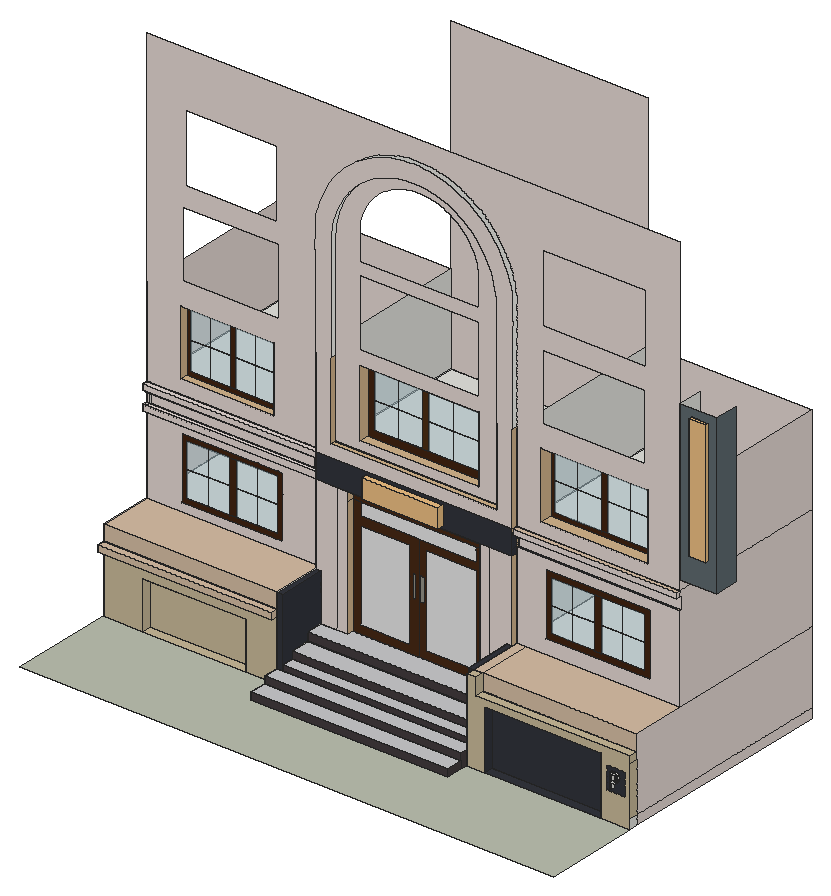
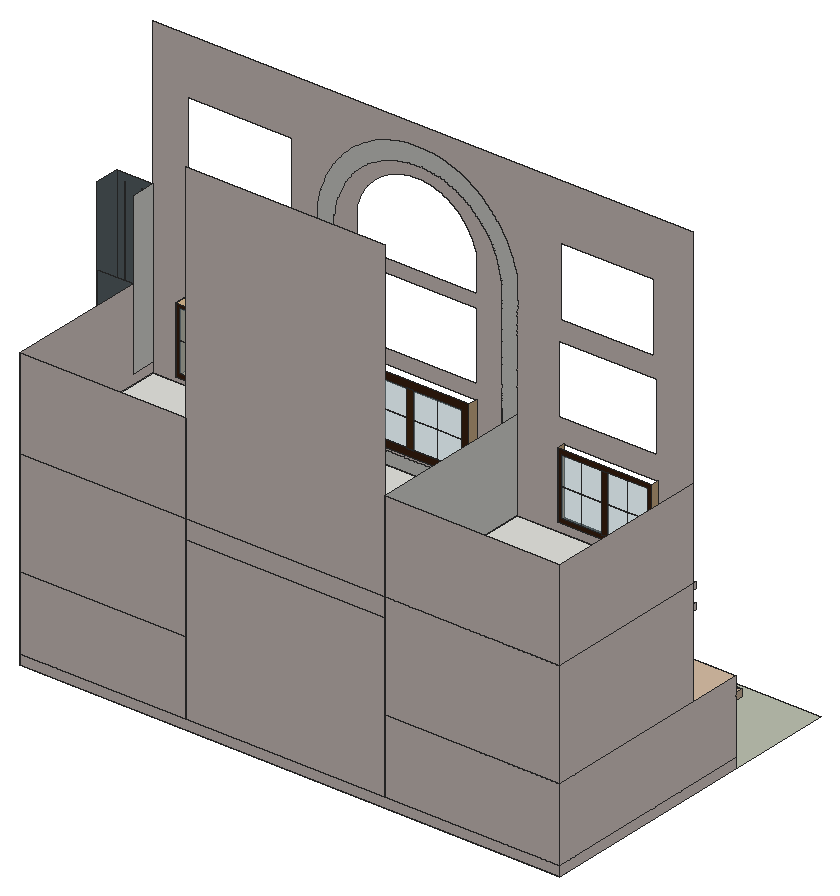
# SketchUp Ruby script. Lengths in inches.
U = 1.inch
M = Sketchup.active_model
def pt(a) = Geom::Point3d.new(a.map { |v| v * U })
def face(e, loops, mat)
  f = e.add_face(loops[0].map { |a| pt(a) })
  loops[1..].each { |l| e.add_face(l.map { |a| pt(a) }).erase! }
  f.material = f.back_material = mat if mat
  f
end
# faces: each face lists its corners as indices into pts; further lists are holes
def faces(e, pts, list, mat = nil) = list.each { |f| face(e, (f[0].is_a?(Array) ? f : [f]).map { |l| l.map { |i| pts[i] } }, mat) }
# xy, xz, yz: faces in a plane at the given z, y or x. An outline is a flat list of corners, or four numbers for a rectangle; further outlines are holes
def ring(l) = l.size == 4 ? [[l[0], l[1]], [l[2], l[1]], [l[2], l[3]], [l[0], l[3]]] : l.each_slice(2).to_a
def flat(e, list, mat, &to3) = list.each { |f| face(e, (f[0].is_a?(Array) ? f : [f]).map { |l| ring(l).map { |u, v| to3.(u, v) } }, mat) }
def xy(e, z, list, mat = nil) = flat(e, list, mat) { |x, y| [x, y, z] }
def xz(e, y, list, mat = nil) = flat(e, list, mat) { |x, z| [x, y, z] }
def yz(e, x, list, mat = nil) = flat(e, list, mat) { |y, z| [x, y, z] }
def lines(e, pts, list) = list.each { |a, b| e.add_line(pt(pts[a]), pt(pts[b])) }
# prism: a flat outline (further loops are holes) pulled along v
def prism(e, loops, v, mat = nil)
  f = face(e, loops, mat); d = Geom::Vector3d.new(v.map { |x| x * U })
  f.pushpull(f.normal.samedirection?(d) ? d.length : -d.length)
end
def box(e, o, s, mat = nil) = prism(e, [[o, [o[0] + s[0], o[1], o[2]], [o[0] + s[0], o[1] + s[1], o[2]], [o[0], o[1] + s[1], o[2]]]], [0, 0, s[2]], mat)
def at(x, y, z, deg = 0) = Geom::Transformation.translation(pt([x, y, z])) * Geom::Transformation.rotation(ORIGIN, Z_AXIS, deg.degrees)
def axes(o, x, y, z) = Geom::Transformation.new([*x, 0, *y, 0, *z, 0, *pt(o).to_a, 1])
def part(name) = M.definitions.add(name)
# library, detail: a bought-in or finely detailed component or shape, given as its bounding box
def library(name, o, s) = part(name).tap { |d| box(d.entities, o, s) }
def detail(e, o, s) = box(e.add_group.entities, o, s)
def put(e, d, t, mat = nil) = e.add_instance(d, t).tap { |i| i.material = mat if mat }
def group(e, t, mat = nil) = e.add_group.tap { |g| g.transformation = t; g.material = mat if mat }.entities
root = M.entities
M.materials.add("[0035_Tan]").color = [210, 180, 140]
M.materials.add("[Asphalt New]").color = [67, 60, 62]
M.materials.add("[Concrete Block 8x8 Gray]").color = [226, 214, 209]
M.materials.add("[Formica Graystone]").color = [149, 146, 135]
M.materials.add("[Formica Laminate Dark]").color = [50, 53, 60]
M.materials.add("[Formica Laminate Light]").color = [213, 189, 164]
M.materials.add("[Formica Speckled Grey]").color = [94, 105, 111]
M.materials.add("[Mirror 02]").color = [229, 229, 229]
M.materials.add("[Pavers with Grass Brick]").color = [187, 192, 176]
M.materials.add("[Polished Concrete New]").color = [200, 200, 203]
M.materials.add("[Quartz Light Brown]").color = [199, 184, 152]
M.materials.add("[Translucent Glass Safety]").color = [204, 235, 244]
M.materials["[Translucent Glass Safety]"].alpha = 0.5
M.materials.add("[Wood Cherry Original]").color = [66, 37, 18]
M.materials.add("[Wood Floor Parquet]").color = [76, 46, 20]
M.materials.add("[Wood Veneer 01]").color = [71, 41, 22]
c1 = part("P")
prism(c1.entities,[[[1.71,0,0],[1.71,9.6,0],[4.83,9.6,0],[6.26,9.52,0],[7.21,9.3,0],[7.85,8.91,0],[8.3,8.38,0],[8.57,7.7,0],[8.66,6.875,0],[8.59,6.16,0],[8.37,5.53,0],[8,4.97,0],[7.49,4.5,0],[6.85,4.13,0],[6.1,3.86,0],[5.23,3.7,0],[4.26,3.64,0],[3.18,3.64,0],[3.18,0,0]],[[3.18,4.75,0],[4.1,4.75,0],[5.41,4.88,0],[5.92,5.05,0],[6.34,5.27,0],[6.67,5.57,0],[6.91,5.93,0],[7.05,6.35,0],[7.09,6.85,0],[6.95,7.6,0],[6.77,7.89,0],[6.53,8.11,0],[5.77,8.4,0],[4.65,8.49,0],[3.18,8.49,0]]],[0,0,12])
c2 = library("HOTEL\#1",[2.3,0,0],[71.65,18.15,12])
c3 = library("H O T E L\#3",[0.1875,0,0],[9.27,75.16,12])
xy(root,0,[[178.17,67.12,363.16,83.17],[178.17,83.17,363.16,97.98],[363.16,89.54,380.11,97.98],[489.41,89.54,516.88,97.98],[15.125,97.98,15.125,302.95,516.88,302.95,516.88,97.98,148.51,97.98,148.51,106.6,51.82,106.6,51.82,97.98]])
xy(root,0,[[380.11,89.54,489.41,97.98]],"[Formica Laminate Dark]")
xy(root,0,[[15.125,0,15.125,97.98,178.17,97.98,178.17,67.12,363.16,67.12,363.16,89.54,516.88,89.54,516.88,0]],"[Pavers with Grass Brick]")
xy(root,0,[[51.82,97.98,148.51,106.6]],"[Quartz Light Brown]")
xy(root,7,[[178.17,67.12,363.16,83.17]],"[Polished Concrete New]")
xy(root,9,[[178.17,97.98,183.48,121.18],[358.34,97.98,363.16,121.18],[183.48,109.36,183.48,121.18,178.17,121.18,178.17,144.37,363.16,144.37,363.16,121.18,358.34,121.18,358.34,109.36],[178.17,144.37,363.16,166.65],[178.17,166.65,363.16,190.35],
  [178.17,190.35,363.16,216.4375],[178.17,216.4375,363.16,239.12],[178.17,239.12,363.16,302.95]])
xy(root,13.1875,[[178.17,83.17,363.16,97.98]],"[Polished Concrete New]")
xy(root,15,[[178.17,121.18,183.48,144.37],[358.34,121.18,363.16,144.37],[183.48,127.56,358.34,144.37]])
xy(root,18.1875,[[183.48,97.98,358.34,109.36]],"[Polished Concrete New]")
xy(root,20.75,[[178.17,144.37,183.48,166.65],[358.34,144.37,363.16,166.65],[183.48,148.73,358.34,166.65]])
xy(root,24.9375,[[183.48,109.36,358.34,127.56]],"[Polished Concrete New]")
xy(root,27.6875,[[178.17,166.65,183.48,190.35],[358.34,166.65,363.16,190.35]])
xy(root,33.1875,[[183.48,143.23,198.71,148.73],[198.71,143.23,208.74,148.73],[332.39,143.23,341.41,148.73],[341.41,143.23,358.34,148.73]])
xy(root,33.1875,[[183.48,127.56,358.34,127.56,358.34,143.23,332.39,143.23,332.39,148.73,208.74,148.73,208.74,143.23,183.48,143.23]],"[Polished Concrete New]")
xy(root,35.125,[[178.17,190.35,183.48,216.4375],[358.34,190.35,363.16,216.4375]])
xy(root,44.5,[[178.17,216.4375,183.48,239.12],[358.34,216.4375,363.16,239.12]])
xy(root,44.6875,[[51.82,97.98,148.51,106.6]],"[Quartz Light Brown]")
xy(root,55.22,[[380.11,89.54,489.41,97.98]],"[Formica Laminate Dark]")
xy(root,56.6,[[15.125,91.54,178.17,97.98]])
xy(root,62.03,[[371.625,89.54,516.88,97.98]],"[Quartz Light Brown]")
xy(root,63.14,[[15.125,91.54,178.17,97.98]],"[Formica Laminate Light]")
xy(root,77.375,[[178.17,143.23,183.48,239.12],[358.34,143.23,363.16,239.12],[15.125,148.73,178.17,302.95],[363.16,148.73,516.88,302.95]])
xy(root,77.375,[[178.17,97.98,183.48,143.23],[358.34,97.98,363.16,143.23]],"[Formica Laminate Dark]")
xy(root,77.375,[[15.125,97.98,178.17,148.73],[363.16,97.98,371.625,148.73],[371.625,97.98,516.88,148.73]],"[Formica Laminate Light]")
xy(root,77.375,[[363.16,89.54,371.625,97.98]],"[Quartz Light Brown]")
xy(root,152.83,[[178.17,143.23,198.71,148.17],[198.71,143.23,208.74,148.17],[332.39,143.23,341.41,148.17],[341.41,143.23,363.16,148.17],[178.17,148.17,198.71,148.73],
  [198.71,148.17,208.74,148.73],[208.74,148.17,332.39,148.73],[332.39,148.17,341.41,148.73],[341.41,148.17,363.16,148.73]])
xy(root,152.83,[[15.125,144.35,178.17,148.73]],"[Concrete Block 8x8 Gray]")
xy(root,152.83,[[208.74,143.23,332.39,148.17]],"[Formica Laminate Dark]")
xy(root,158.16,[[173.28,144.35,178.17,148.73]])
xy(root,158.16,[[15.125,144.35,18.04,148.73],[18.04,144.35,173.28,148.73],[18.04,148.73,173.28,149.6]],"[Concrete Block 8x8 Gray]")
xy(root,158.3125,[[363.16,148.73,516.88,150.98]],"[Formica Laminate Light]")
xy(root,170.03,[[173.28,144.35,178.17,148.73]])
xy(root,170.03,[[15.125,144.35,18.04,148.73],[18.04,144.35,173.28,148.73],[18.04,148.73,173.28,149.6]],"[Concrete Block 8x8 Gray]")
xy(root,170.13,[[363.16,144.54,516.88,148.73],[363.16,148.73,516.88,150.98]],"[Formica Laminate Light]")
xy(root,175.6875,[[178.17,143.23,363.16,148.17],[178.17,148.17,363.16,148.73],[15.125,148.73,178.17,302.95],[178.17,148.73,363.16,302.95],[363.16,148.73,516.88,302.95]])
xy(root,175.6875,[[15.125,144.35,178.17,148.73]],"[Concrete Block 8x8 Gray]")
xy(root,175.6875,[[363.16,144.54,516.88,148.73]],"[Formica Laminate Light]")
xy(root,184.73,[[516.88,148.73,550.94,171.42]],"[Formica Speckled Grey]")
xy(root,187.27,[[192.26,143.23,349.07,148.73]],"[0035_Tan]")
xy(root,187.57,[[386.1,148.73,486.62,159.67]],"[0035_Tan]")
xy(root,188.76,[[47.15,148.73,134.71,155.98]],"[0035_Tan]")
xy(root,196.03,[[215.4,148.73,327.53,158.04]],"[0035_Tan]")
xy(root,249.7,[[386.1,148.73,486.62,159.67]],"[0035_Tan]")
xz(root,67.12,[[178.17,0,363.16,7]],"[Asphalt New]")
xz(root,83.17,[[178.17,0,363.16,7]])
xz(root,83.17,[[178.17,7,363.16,13.1875]],"[Asphalt New]")
xz(root,89.54,[[495.2,25.96,512.01,46.65]],"[Formica Laminate Dark]")
xz(root,89.54,[[[363.16,0,380.11,0,380.11,55.22,489.41,55.22,489.41,0,516.88,0,516.88,62.03,371.625,62.03,371.625,77.375,363.16,77.375],[495.2,25.96,512.01,46.65]]],"[Quartz Light Brown]")
xz(root,91.54,[[15.125,56.6,178.17,63.14]],"[Formica Laminate Light]")
xz(root,97.98,[[178.17,0,178.17,9,183.48,9,183.48,13.1875,358.34,13.1875,358.34,9,363.16,9,363.16,0],[363.16,0,380.11,55.22],[489.41,0,516.88,55.22],[178.17,9,183.48,13.1875],[358.34,9,363.16,13.1875],
  [363.16,55.22,363.16,77.375,371.625,77.375,371.625,62.03,516.88,62.03,516.88,55.22],[15.125,56.6,178.17,63.14]])
xz(root,97.98,[[183.48,13.1875,358.34,18.1875]],"[Asphalt New]")
xz(root,97.98,[[380.11,0,489.41,55.22],[178.17,13.1875,183.48,77.375],[358.34,13.1875,363.16,77.375]],"[Formica Laminate Dark]")
xz(root,97.98,[[371.625,62.03,516.88,77.375],[15.125,63.14,178.17,77.375]],"[Formica Laminate Light]")
xz(root,97.98,[[15.125,0,51.82,0,51.82,44.6875,148.51,44.6875,148.51,0,178.17,0,178.17,56.6,15.125,56.6]],"[Quartz Light Brown]")
xz(root,106.6,[[51.82,0,148.51,44.6875]],"[Quartz Light Brown]")
xz(root,109.36,[[183.48,9,358.34,18.1875]])
xz(root,109.36,[[183.48,18.1875,358.34,24.9375]],"[Asphalt New]")
xz(root,121.18,[[178.17,9,183.48,15],[358.34,9,363.16,15]])
xz(root,127.56,[[183.48,15,358.34,24.9375]])
xz(root,127.56,[[183.48,24.9375,358.34,33.1875]],"[Asphalt New]")
xz(root,143.23,[[183.48,33.1875,198.71,33.1875,198.71,152.83,178.17,152.83,178.17,77.375,183.48,77.375],[198.71,33.1875,208.74,152.83],[332.39,33.1875,341.41,152.83],[341.41,33.1875,358.34,33.1875,358.34,77.375,363.16,77.375,363.16,152.83,341.41,152.83],[[178.17,175.6875,363.16,175.6875,363.16,343.6875,363.18,356.6,363.35,353.85,363.39,348.77,363.16,343.6875,363.16,370.47,362.44,374.86,361.49,379.2,360.34,383.5,358.99,387.74,357.43,391.91,355.68,395.99,353.74,400,351.6,403.9,349.29,407.7,346.8,411.38,344.13,414.94,341.3,418.37,338.3,421.66,335.16,424.81,331.87,427.8,328.4375,430.63,324.875,433.3,321.19,435.79,317.39,438.11,313.49,440.24,309.49,442.18,305.4,443.93,301.23,445.49,296.99,446.84,292.7,447.99,288.35,448.9375,283.96,449.67,279.55,450.2,275.11,450.52,270.66,450.625,266.22,450.52,261.78,450.2,257.36,449.67,252.98,448.9375,248.63,447.99,244.33,446.84,240.09,445.49,235.93,443.93,231.84,442.18,227.84,440.24,223.93,438.11,220.13,435.79,216.45,433.3,212.89,430.63,209.46,427.8,206.17,424.81,203.02,421.66,200.03,418.37,197.2,414.94,194.53,411.38,192.04,407.7,189.72,403.9,187.59,400,185.64,395.99,183.89,391.91,182.34,387.74,180.98,383.5,179.83,379.2,178.88,374.86,178.17,370.47,178.17,343.6875,177.93,348.77,177.97,353.85,178.15,356.6,178.17,343.6875],[192.26,187.27,192.26,356.49,192.36,360.59,192.6875,364.68,193.22,368.75,193.97,372.79,194.93,376.78,196.09,380.72,197.46,384.59,199.03,388.38,200.8,392.08,202.76,395.69,204.91,399.19,207.23,402.57,209.73,405.83,212.4,408.95,215.22,411.93,218.2,414.76,221.32,417.42,224.58,419.92,227.96,422.25,231.46,424.39,235.07,426.35,238.77,428.12,242.5625,429.6875,246.43,431.06,250.37,432.22,254.36,433.18,258.4,433.93,262.47,434.47,266.56,434.79,270.66,434.89,274.77,434.79,278.86,434.47,282.93,433.93,286.96,433.18,290.96,432.22,294.89,431.06,298.76,429.6875,302.55,428.12,306.26,426.35,309.87,424.39,313.37,422.25,316.75,419.92,320.01,417.42,323.13,414.76,326.1,411.93,328.93,408.95,331.6,405.83,334.1,402.57,336.42,399.19,338.56,395.69,340.52,392.08,342.29,388.38,343.86,384.59,345.23,380.72,346.4,376.78,347.36,372.79,348.1,368.75,348.64,364.68,348.96,360.59,349.07,356.49,349.07,187.27]]],"[Concrete Block 8x8 Gray]")
xz(root,143.23,[[178.17,152.83,363.16,175.6875]],"[Formica Laminate Dark]")
xz(root,144.35,[[15.125,152.83,178.17,158.16],[15.125,170.03,178.17,175.6875]],"[Concrete Block 8x8 Gray]")
xz(root,144.37,[[178.17,9,363.16,15],[178.17,15,183.48,20.75],[358.34,15,363.16,20.75]])
xz(root,144.54,[[363.16,170.13,516.88,175.6875]],"[Concrete Block 8x8 Gray]")
xz(root,148.17,[[178.17,152.83,363.16,175.6875]])
xz(root,148.73,[[183.48,20.75,358.34,33.1875],[15.125,152.83,178.17,158.16],[178.17,152.83,363.16,175.6875],[15.125,170.03,178.17,175.6875],[363.16,170.13,516.88,175.6875],
  [[178.17,175.6875,178.17,343.6875,178.15,356.6,177.97,353.85,177.93,348.77,178.17,343.6875,178.17,370.47,178.88,374.86,179.83,379.2,180.98,383.5,182.34,387.74,183.89,391.91,185.64,395.99,187.59,400,189.72,403.9,192.04,407.7,194.53,411.38,197.2,414.94,200.03,418.37,203.02,421.66,206.17,424.81,209.46,427.8,212.89,430.63,216.45,433.3,220.13,435.79,223.93,438.11,227.84,440.24,231.84,442.18,235.93,443.93,240.09,445.49,244.33,446.84,248.63,447.99,252.98,448.9375,257.36,449.67,261.78,450.2,266.22,450.52,270.66,450.625,275.11,450.52,279.55,450.2,283.96,449.67,288.35,448.9375,292.7,447.99,296.99,446.84,301.23,445.49,305.4,443.93,309.49,442.18,313.49,440.24,317.39,438.11,321.19,435.79,324.875,433.3,328.4375,430.63,331.87,427.8,335.16,424.81,338.3,421.66,341.3,418.37,344.13,414.94,346.8,411.38,349.29,407.7,351.6,403.9,353.74,400,355.68,395.99,357.43,391.91,358.99,387.74,360.34,383.5,361.49,379.2,362.44,374.86,363.16,370.47,363.16,343.6875,363.39,348.77,363.35,353.85,363.18,356.6,363.16,343.6875,363.16,175.6875],[192.26,187.27,349.07,187.27,349.07,356.49,348.96,360.59,348.64,364.68,348.1,368.75,347.36,372.79,346.4,376.78,345.23,380.72,343.86,384.59,342.29,388.38,340.52,392.08,338.56,395.69,336.42,399.19,334.1,402.57,331.6,405.83,328.93,408.95,326.1,411.93,323.13,414.76,320.01,417.42,316.75,419.92,313.37,422.25,309.87,424.39,306.26,426.35,302.55,428.12,298.76,429.6875,294.89,431.06,290.96,432.22,286.96,433.18,282.93,433.93,278.86,434.47,274.77,434.79,270.66,434.89,266.56,434.79,262.47,434.47,258.4,433.93,254.36,433.18,250.37,432.22,246.43,431.06,242.5625,429.6875,238.77,428.12,235.07,426.35,231.46,424.39,227.96,422.25,224.58,419.92,221.32,417.42,218.2,414.76,215.22,411.93,212.4,408.95,209.73,405.83,207.23,402.57,204.91,399.19,202.76,395.69,200.8,392.08,199.03,388.38,197.46,384.59,196.09,380.72,194.93,376.78,193.97,372.79,193.22,368.75,192.6875,364.68,192.36,360.59,192.26,356.49]]])
xz(root,148.73,[[[15.125,77.375,178.17,152.83],[48.4,85.19,143.36,143.88]],[[363.16,77.375,516.88,158.3125],[390.21,90.58,488.96,149.4]],[15.125,158.16,18.04,170.03],[173.28,158.16,178.17,170.03],[[15.125,175.6875,178.17,175.6875,178.17,343.6875,177.93,348.77,177.97,353.85,178.15,356.6,178.125,370.32,178.17,370.47,178.88,374.86,179.83,379.2,180.98,383.5,182.34,387.74,183.89,391.91,185.64,395.99,187.59,400,189.72,403.9,192.04,407.7,194.53,411.38,197.2,414.94,200.03,418.37,203.02,421.66,206.17,424.81,209.46,427.8,212.89,430.63,216.45,433.3,220.13,435.79,223.93,438.11,227.84,440.24,231.84,442.18,235.93,443.93,240.09,445.49,244.33,446.84,248.63,447.99,252.98,448.9375,257.36,449.67,261.78,450.2,266.22,450.52,270.66,450.625,275.11,450.52,279.55,450.2,283.96,449.67,288.35,448.9375,292.7,447.99,296.99,446.84,301.23,445.49,305.4,443.93,309.49,442.18,313.49,440.24,317.39,438.11,321.19,435.79,324.875,433.3,328.4375,430.63,331.87,427.8,335.16,424.81,338.3,421.66,341.3,418.37,344.13,414.94,346.8,411.38,349.29,407.7,351.6,403.9,353.74,400,355.68,395.99,357.43,391.91,358.99,387.74,360.34,383.5,361.49,379.2,362.44,374.86,363.16,370.47,363.2,370.32,363.18,356.6,363.35,353.85,363.39,348.77,363.16,343.6875,363.16,175.6875,516.88,175.6875,516.88,469.3125,15.125,469.3125],[387.3,352.68,484.24,417.24],[386.1,187.57,486.62,249.7],[387.81,270.29,483.43,332.73],[48.61,271.61,139.11,334.67],[51.46,352.89,137.53,417.08],[47.15,188.76,134.71,250.26]],
  [[192.26,187.27,349.07,187.27,349.07,356.49,348.96,360.59,348.64,364.68,348.1,368.75,347.36,372.79,346.4,376.78,345.23,380.72,343.86,384.59,342.29,388.38,340.52,392.08,338.56,395.69,336.42,399.19,334.1,402.57,331.6,405.83,328.93,408.95,326.1,411.93,323.13,414.76,320.01,417.42,316.75,419.92,313.37,422.25,309.87,424.39,306.26,426.35,302.55,428.12,298.76,429.6875,294.89,431.06,290.96,432.22,286.96,433.18,282.93,433.93,278.86,434.47,274.77,434.79,270.66,434.89,266.56,434.79,262.47,434.47,258.4,433.93,254.36,433.18,250.37,432.22,246.43,431.06,242.5625,429.6875,238.77,428.12,235.07,426.35,231.46,424.39,227.96,422.25,224.58,419.92,221.32,417.42,218.2,414.76,215.22,411.93,212.4,408.95,209.73,405.83,207.23,402.57,204.91,399.19,202.76,395.69,200.8,392.08,199.03,388.38,197.46,384.59,196.09,380.72,194.93,376.78,193.97,372.79,193.22,368.75,192.6875,364.68,192.36,360.59,192.26,356.49],[215.4,346.9,215.4,378.59,215.98,381.14,216.68,383.65,217.49,386.14,218.41,388.58,219.44,390.98,220.58,393.33,221.83,395.63,223.18,397.86,224.63,400.04,226.18,402.14,227.82,404.17,229.56,406.125,231.38,408,233.28,409.79,235.27,411.48,237.33,413.09,239.46,414.6,241.66,416.01,243.92,417.32,246.24,418.53,248.61,419.625,251.03,420.61,253.49,421.49,255.99,422.26,258.52,422.91,261.07,423.4375,263.65,423.85,266.25,424.15,268.85,424.33,271.47,424.39,274.08,424.33,276.68,424.15,279.28,423.85,281.86,423.4375,284.42,422.91,286.95,422.26,289.44,421.49,291.91,420.61,294.32,419.625,296.69,418.53,299.01,417.32,301.27,416.01,303.47,414.6,305.6,413.09,307.66,411.48,309.65,409.79,311.55,408,313.375,406.125,315.11,404.17,316.75,402.14,318.3,400.04,319.75,397.86,321.1,395.63,322.35,393.33,323.49,390.98,324.52,388.58,325.44,386.14,326.25,383.65,326.95,381.14,327.53,378.59,327.53,346.9],[215.4,196.03,327.53,259.4],[215.4,272.4,327.53,335.78]]],"[Concrete Block 8x8 Gray]")
xz(root,148.73,[[265.13,80.19,268.07,102],[272.95,80.19,275.88,102]],"[Formica Graystone]")
xz(root,148.73,[[516.88,184.73,550.94,332.73]],"[Formica Speckled Grey]")
xz(root,148.73,[[216.49,40.94,262.81,124.79],[278.32,40.94,324.63,124.79],[216.49,132.55,324.63,144.83]],"[Mirror 02]")
xz(root,148.73,[[53.22,90.01,73.1875,114.54],[73.1875,90.01,93.16,114.54],[99.71,90.01,119.125,114.54],[119.125,90.01,138.54,114.54],[395.91,96.28,416.09,119.99],
  [416.09,96.28,436.27,119.99],[442.69,96.28,462.97,119.99],[462.97,96.28,483.26,119.99],[53.22,114.54,73.1875,139.0625],[73.1875,114.54,93.16,139.0625],
  [99.71,114.54,119.125,139.0625],[119.125,114.54,138.54,139.0625],[395.91,119.99,416.09,143.7],[416.09,119.99,436.27,143.7],[442.69,119.99,462.97,143.7],
  [462.97,119.99,483.26,143.7]],"[Translucent Glass Safety]")
xz(root,148.73,[[[48.4,85.19,143.36,143.88],[53.22,90.01,138.54,139.0625]],[93.16,90.01,99.71,139.0625],[[390.21,90.58,488.96,149.4],[395.91,96.28,483.26,143.7]],[436.27,96.28,442.69,143.7]],"[Wood Cherry Original]")
xz(root,148.73,[[[208.74,33.1875,270.56,33.1875,270.56,132.55,216.49,132.55,216.49,124.79,262.81,124.79,262.81,40.94,216.49,40.94,216.49,144.83,208.74,144.83],[265.13,80.19,268.07,102]],[[270.56,33.1875,332.39,33.1875,332.39,144.83,324.63,144.83,324.63,40.94,278.32,40.94,278.32,124.79,324.63,124.79,324.63,132.55,270.56,132.55],[272.95,80.19,275.88,102]],[208.74,144.83,332.39,152.83]],"[Wood Veneer 01]")
xz(root,149.6,[[18.04,158.16,173.28,170.03]],"[Concrete Block 8x8 Gray]")
xz(root,150.98,[[363.16,158.3125,516.88,170.13]],"[Concrete Block 8x8 Gray]")
xz(root,155.98,[[51.14,192.75,69.625,219.51],[69.625,192.75,88.12,219.51],[93.35,192.75,112.04,219.51],[112.04,192.75,130.73,219.51],[51.14,219.51,69.625,246.28],
  [69.625,219.51,88.12,246.28],[93.35,219.51,112.04,246.28],[112.04,219.51,130.73,246.28]],"[Translucent Glass Safety]")
xz(root,155.98,[[[47.15,188.76,134.71,250.26],[51.14,192.75,130.73,246.28]],[88.12,192.75,93.35,246.28]],"[Wood Cherry Original]")
xz(root,158.04,[[222.14,202.76,244.65,227.71],[244.65,202.76,267.17,227.71],[272.89,202.76,296.84,227.71],[296.84,202.76,320.79,227.71],[222.14,227.71,244.65,252.66],
  [244.65,227.71,267.17,252.66],[272.89,227.71,296.84,252.66],[296.84,227.71,320.79,252.66]],"[Translucent Glass Safety]")
xz(root,158.04,[[[215.4,196.03,327.53,259.4],[222.14,202.76,320.79,252.66]]],"[Wood Cherry Original]")
xz(root,158.04,[[267.17,202.76,272.89,252.66]],"[Wood Floor Parquet]")
xz(root,159.67,[[389.75,191.22,412.22,218.64],[412.22,191.22,434.69,218.64],[440.03,191.22,461.51,218.64],[461.51,191.22,482.98,218.64],[389.75,218.64,412.22,246.06],
  [412.22,218.64,434.69,246.06],[440.03,218.64,461.51,246.06],[461.51,218.64,482.98,246.06]],"[Translucent Glass Safety]")
xz(root,159.67,[[[386.1,187.57,486.62,249.7],[389.75,191.22,482.98,246.06]],[434.69,191.22,440.03,246.06]],"[Wood Cherry Original]")
xz(root,166.65,[[178.17,9,363.16,20.75],[178.17,20.75,183.48,27.6875],[358.34,20.75,363.16,27.6875]])
xz(root,171.42,[[516.88,184.73,550.94,259.6875]],"[Formica Speckled Grey]")
xz(root,190.35,[[178.17,9,363.16,27.6875],[178.17,27.6875,183.48,35.125],[358.34,27.6875,363.16,35.125]])
xz(root,216.4375,[[178.17,9,363.16,35.125],[178.17,35.125,183.48,44.5],[358.34,35.125,363.16,44.5]])
xz(root,239.12,[[178.17,9,363.16,44.5],[178.17,44.5,183.48,77.375],[358.34,44.5,363.16,77.375]])
xz(root,302.95,[[15.125,0,516.88,9],[15.125,9,178.17,77.375],[178.17,9,363.16,158.3125],[363.16,9,516.88,77.375],[15.125,77.375,178.17,175.6875],
  [363.16,77.375,516.88,175.6875],[178.17,158.3125,363.16,175.6875],[15.125,175.6875,178.17,259.6875],[178.17,175.6875,363.16,469.3125],[363.16,175.6875,516.88,259.6875]],"[Concrete Block 8x8 Gray]")
yz(root,15.125,[[97.98,0,302.95,9],[97.98,9,302.95,77.375],[148.73,77.375,302.95,175.6875],[144.35,152.83,148.73,158.16],[144.35,170.03,148.73,175.6875],
  [148.73,175.6875,302.95,259.6875]],"[Concrete Block 8x8 Gray]")
yz(root,15.125,[[91.54,56.6,97.98,63.14]],"[Formica Laminate Light]")
yz(root,18.04,[[148.73,158.16,149.6,170.03]])
yz(root,47.15,[[148.73,188.76,155.98,250.26]],"[0035_Tan]")
yz(root,51.82,[[97.98,0,106.6,44.6875]],"[Quartz Light Brown]")
yz(root,134.71,[[148.73,188.76,155.98,250.26]],"[0035_Tan]")
yz(root,148.51,[[97.98,0,106.6,44.6875]],"[Quartz Light Brown]")
yz(root,173.28,[[148.73,158.16,149.6,170.03]])
yz(root,178.17,[[97.98,9,97.98,77.375,239.12,77.375,239.12,44.5,216.4375,44.5,216.4375,35.125,190.35,35.125,190.35,27.6875,166.65,27.6875,166.65,20.75,144.37,20.75,144.37,15,121.18,15,121.18,9],[121.18,9,144.37,15],[144.37,9,166.65,20.75],[166.65,9,190.35,27.6875],[190.35,9,216.4375,35.125],
  [216.4375,9,239.12,44.5],[239.12,9,302.95,77.375],[148.73,77.375,302.95,158.3125],[143.23,152.83,144.35,158.16],[144.35,152.83,148.17,158.16],
  [148.17,152.83,148.73,158.16],[143.23,158.16,148.17,158.3125],[148.17,158.16,148.73,158.3125],[148.17,158.3125,148.73,170.03],[148.73,158.3125,302.95,175.6875],
  [143.23,170.03,144.35,175.6875],[144.35,170.03,148.17,175.6875],[148.17,170.03,148.73,175.6875],[148.73,175.6875,302.95,259.6875]])
yz(root,178.17,[[143.23,77.375,148.73,152.83],[143.23,175.6875,148.73,259.6875]],"[0035_Tan]")
yz(root,178.17,[[67.12,0,83.17,7],[83.17,0,97.98,13.1875]],"[Asphalt New]")
yz(root,178.17,[[143.23,158.3125,148.17,170.03]],"[Formica Laminate Dark]")
yz(root,178.17,[[91.54,56.6,97.98,63.14]],"[Formica Laminate Light]")
yz(root,183.48,[[97.98,9,109.36,18.1875],[109.36,9,121.18,24.9375],[121.18,15,127.56,24.9375],[127.56,15,144.37,33.1875],[144.37,20.75,148.73,33.1875],
  [148.73,20.75,166.65,27.6875],[148.73,27.6875,190.35,27.6875,190.35,35.125,143.23,35.125,143.23,33.1875,148.73,33.1875],[143.23,35.125,216.4375,44.5],[143.23,44.5,239.12,77.375]])
yz(root,183.48,[[97.98,18.1875,109.36,18.1875,109.36,24.9375,127.56,24.9375,127.56,33.1875,143.23,33.1875,143.23,77.375,97.98,77.375]],"[Formica Laminate Dark]")
yz(root,192.26,[[143.23,187.27,148.73,259.6875]],"[0035_Tan]")
yz(root,208.74,[[143.23,33.1875,148.73,144.83],[143.23,144.83,148.73,152.83]],"[0035_Tan]")
yz(root,215.4,[[148.73,196.03,158.04,259.4]],"[0035_Tan]")
yz(root,327.53,[[148.73,196.03,158.04,259.4]],"[0035_Tan]")
yz(root,332.39,[[143.23,33.1875,148.73,144.83],[143.23,144.83,148.73,152.83]],"[0035_Tan]")
yz(root,349.07,[[143.23,187.27,148.73,259.6875]])
yz(root,358.34,[[97.98,9,109.36,18.1875],[109.36,9,121.18,24.9375],[121.18,15,127.56,24.9375],[127.56,15,144.37,33.1875],[144.37,20.75,148.73,33.1875],
  [148.73,20.75,166.65,27.6875],[148.73,27.6875,148.73,33.1875,143.23,33.1875,143.23,35.125,190.35,35.125,190.35,27.6875],[143.23,35.125,216.4375,44.5],[143.23,44.5,239.12,77.375]])
yz(root,358.34,[[97.98,18.1875,97.98,77.375,143.23,77.375,143.23,33.1875,127.56,33.1875,127.56,24.9375,109.36,24.9375,109.36,18.1875]],"[Formica Laminate Dark]")
yz(root,363.16,[[89.54,0,97.98,9],[89.54,9,97.98,13.1875],[97.98,9,121.18,9,121.18,15,144.37,15,144.37,20.75,166.65,20.75,166.65,27.6875,190.35,27.6875,190.35,35.125,216.4375,35.125,216.4375,44.5,239.12,44.5,239.12,77.375,97.98,77.375],[121.18,9,144.37,15],[144.37,9,166.65,20.75],
  [166.65,9,190.35,27.6875],[190.35,9,216.4375,35.125],[216.4375,9,239.12,44.5],[239.12,9,302.95,77.375],[148.73,77.375,302.95,158.3125],
  [148.17,152.83,148.73,158.3125],[150.98,158.3125,150.98,170.13,148.73,170.13,148.73,175.6875,302.95,175.6875,302.95,158.3125],[144.54,170.13,148.17,175.6875],[148.17,170.13,148.73,175.6875],[148.73,175.6875,302.95,259.6875]])
yz(root,363.16,[[143.23,77.375,148.73,152.83],[148.17,158.3125,148.73,170.13],[148.73,158.3125,150.98,170.13],[143.23,170.13,144.54,175.6875],[143.23,175.6875,148.73,259.6875]],"[0035_Tan]")
yz(root,363.16,[[67.12,0,83.17,7],[83.17,0,89.54,13.1875]],"[Asphalt New]")
yz(root,363.16,[[143.23,152.83,148.17,158.3125],[143.23,158.3125,148.17,170.13]],"[Formica Laminate Dark]")
yz(root,363.16,[[89.54,13.1875,97.98,55.22],[89.54,55.22,97.98,77.375]],"[Quartz Light Brown]")
yz(root,371.625,[[89.54,62.03,97.98,77.375]],"[Quartz Light Brown]")
yz(root,380.11,[[89.54,0,97.98,55.22]],"[Formica Laminate Dark]")
yz(root,386.1,[[148.73,187.57,159.67,249.7]],"[0035_Tan]")
yz(root,486.62,[[148.73,187.57,159.67,249.7]],"[0035_Tan]")
yz(root,489.41,[[89.54,0,97.98,55.22]],"[Formica Laminate Dark]")
yz(root,516.88,[[89.54,0,97.98,9],[148.73,184.73,171.42,332.73]])
yz(root,516.88,[[97.98,0,302.95,9],[97.98,9,302.95,77.375],[148.73,77.375,302.95,77.375,302.95,175.6875,148.73,175.6875,148.73,170.13,150.98,170.13,150.98,158.3125,148.73,158.3125],[144.54,170.13,148.73,175.6875],[148.73,175.6875,302.95,175.6875,302.95,259.6875,171.42,259.6875,171.42,184.73,148.73,184.73]],"[Concrete Block 8x8 Gray]")
yz(root,516.88,[[89.54,9,97.98,55.22],[89.54,55.22,97.98,62.03]],"[Quartz Light Brown]")
yz(root,550.94,[[148.73,184.73,171.42,332.73]],"[Formica Speckled Grey]")
put(root,c1,axes([498.32,89.54,29.84],[1,0,0],[0,0,1.4375],[0,-0.19,0]))
put(root,c2,axes([223.62,143.23,155.16],[1,0,0],[0,0,1],[0,-0.44,0]))
put(root,c3,axes([527.09,148.73,209.84],[1.7,0,0],[0,0,1.539],[0,-0.26,0]))
